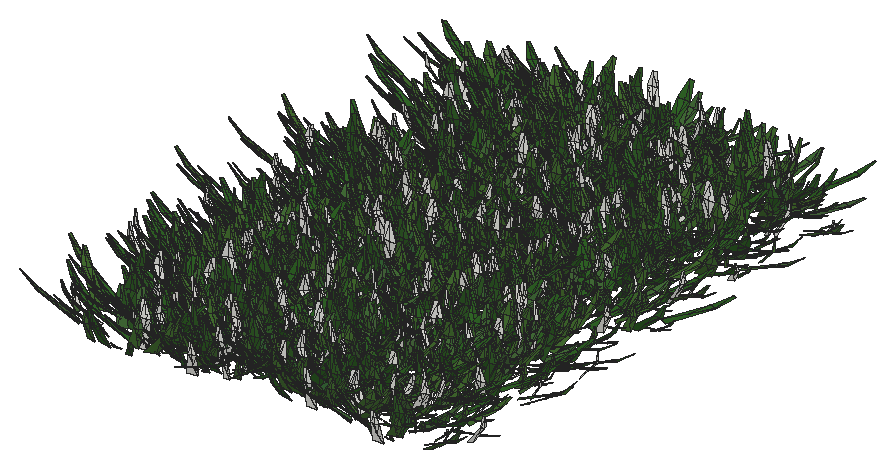
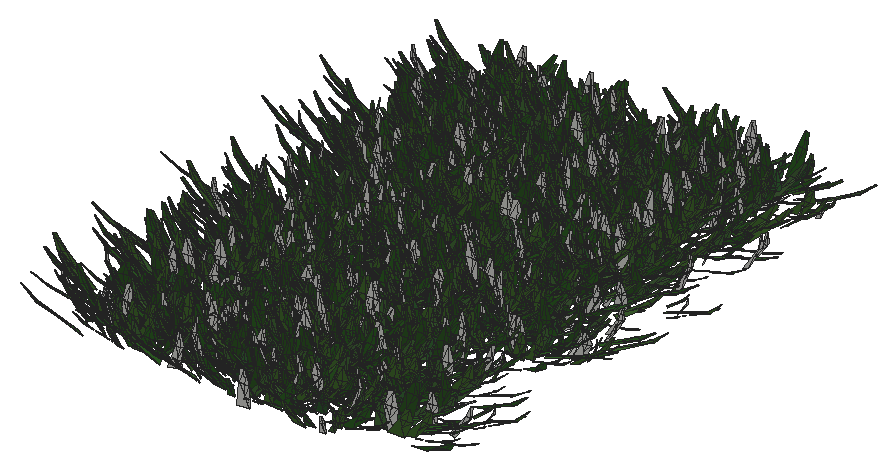
# SketchUp Ruby script. Lengths in inches.
U = 1.inch
M = Sketchup.active_model
def pt(a) = Geom::Point3d.new(a.map { |v| v * U })
def face(e, loops, mat)
  f = e.add_face(loops[0].map { |a| pt(a) })
  loops[1..].each { |l| e.add_face(l.map { |a| pt(a) }).erase! }
  f.material = f.back_material = mat if mat
  f
end
# faces: each face lists its corners as indices into pts; further lists are holes
def faces(e, pts, list, mat = nil) = list.each { |f| face(e, (f[0].is_a?(Array) ? f : [f]).map { |l| l.map { |i| pts[i] } }, mat) }
# xy, xz, yz: faces in a plane at the given z, y or x. An outline is a flat list of corners, or four numbers for a rectangle; further outlines are holes
def ring(l) = l.size == 4 ? [[l[0], l[1]], [l[2], l[1]], [l[2], l[3]], [l[0], l[3]]] : l.each_slice(2).to_a
def flat(e, list, mat, &to3) = list.each { |f| face(e, (f[0].is_a?(Array) ? f : [f]).map { |l| ring(l).map { |u, v| to3.(u, v) } }, mat) }
def xy(e, z, list, mat = nil) = flat(e, list, mat) { |x, y| [x, y, z] }
def xz(e, y, list, mat = nil) = flat(e, list, mat) { |x, z| [x, y, z] }
def yz(e, x, list, mat = nil) = flat(e, list, mat) { |y, z| [x, y, z] }
def lines(e, pts, list) = list.each { |a, b| e.add_line(pt(pts[a]), pt(pts[b])) }
# prism: a flat outline (further loops are holes) pulled along v
def prism(e, loops, v, mat = nil)
  f = face(e, loops, mat); d = Geom::Vector3d.new(v.map { |x| x * U })
  f.pushpull(f.normal.samedirection?(d) ? d.length : -d.length)
end
def box(e, o, s, mat = nil) = prism(e, [[o, [o[0] + s[0], o[1], o[2]], [o[0] + s[0], o[1] + s[1], o[2]], [o[0], o[1] + s[1], o[2]]]], [0, 0, s[2]], mat)
def at(x, y, z, deg = 0) = Geom::Transformation.translation(pt([x, y, z])) * Geom::Transformation.rotation(ORIGIN, Z_AXIS, deg.degrees)
def axes(o, x, y, z) = Geom::Transformation.new([*x, 0, *y, 0, *z, 0, *pt(o).to_a, 1])
def part(name) = M.definitions.add(name)
# library, detail: a bought-in or finely detailed component or shape, given as its bounding box
def library(name, o, s) = part(name).tap { |d| box(d.entities, o, s) }
def detail(e, o, s) = box(e.add_group.entities, o, s)
def put(e, d, t, mat = nil) = e.add_instance(d, t).tap { |i| i.material = mat if mat }
def group(e, t, mat = nil) = e.add_group.tap { |g| g.transformation = t; g.material = mat if mat }.entities
root = M.entities
M.materials.add("Material82").color = [68, 110, 58]
M.materials.add("Material83").color = [48, 90, 38]
M.materials.add("Material84").color = [68, 110, 48]
M.materials.add("Material85").color = [48, 90, 48]
M.materials.add("Material86").color = [58, 110, 58]
M.materials.add("Material87").color = [58, 90, 38]
M.materials.add("Material88").color = [68, 100, 58]
M.materials.add("Material89").color = [48, 100, 38]
c1 = part("grass00")
p = [[-0.6875,0.15,0],[-0.56,0.08,5.52],[-0.04,0.03,2.76],[0.48,-0.02,0],[0.35,-0.02,5.52],[-0.1,-0.14,5.52],
  [-0.12,0.65,8.37],[-0.42,0.65,8.37]]
faces(c1.entities,p,[[0,1,2,3],[3,2,4],[1,5,2],[5,4,2],[1,6,5],[4,5,6],[7,6,1]])
c2 = part("Group16\#1")
put(c2.entities,c1,axes([1.44,-0.61,-0.01],[0.05352,0.12609,0],[-0.10704,0.04543,0.07239],[0.06664,-0.02828,0.11628]),"Material85")
put(c2.entities,c1,axes([0.76,-0.15,-0.01],[0.04676,0.24062,0],[-0.23162,0.04501,0.06642],[0.0652,-0.01267,0.23595]),"Material82")
put(c2.entities,c1,axes([0.79,0.01,-0.01],[-0.00606,0.34651,0],[-0.34381,-0.00602,0.0432],[0.04319,0.00076,0.34386]))
put(c2.entities,c1,axes([1,0.23,-0.01],[-0.07192,0.31144,0],[-0.28722,-0.06632,0.1236],[0.12043,0.02781,0.29478]),"Material84")
put(c2.entities,c1,axes([1.66,0.77,-0.01],[-0.13828,0.29651,0],[-0.21551,-0.1005,0.22471],[0.20365,0.09498,0.23779]),"Material89")
put(c2.entities,c1,axes([0.6875,0.52,-0.01],[-0.18126,0.24051,0],[-0.22746,-0.17142,0.09788],[0.07817,0.05891,0.28481]),"Material84")
put(c2.entities,c1,axes([0.68,0.78,-0.01],[-0.215,0.18688,0],[-0.12385,-0.14248,0.21334],[0.13995,0.16101,0.18878]),"Material82")
put(c2.entities,c1,axes([0.56,1,-0.01],[-0.13756,0.07624,0],[-0.06159,-0.11112,0.0927],[0.04494,0.08108,0.12705]),"Material84")
put(c2.entities,c1,axes([0.2,0.64,-0.01],[-0.23729,0.07254,0],[-0.05711,-0.18681,0.153],[0.04473,0.14632,0.19535]),"Material89")
put(c2.entities,c1,axes([0.0625,0.72,-0.01],[-0.28874,0.02525,0],[-0.02179,-0.24916,0.14647],[0.01276,0.14591,0.25012]),"Material82")
put(c2.entities,c1,axes([-0.08,0.62,-0.01],[-0.34089,-0.04187,0],[0.03255,-0.26504,0.216],[-0.02633,0.21439,0.26703]),"Material89")
put(c2.entities,c1,axes([-0.34,0.98,-0.01],[-0.14314,-0.0493,0],[0.04397,-0.12769,0.06843],[-0.02228,0.0647,0.13505]),"Material89")
put(c2.entities,c1,axes([-0.87,1.45,-0.01],[-0.23488,-0.14114,0],[0.13761,-0.22901,0.06087],[-0.03135,0.05217,0.26717]))
put(c2.entities,c1,axes([-0.72,0.77,-0.01],[-0.14208,-0.13251,0],[0.07209,-0.0773,0.16301],[-0.11118,0.11922,0.1057]),"Material89")
put(c2.entities,c1,axes([-0.62,0.43,-0.01],[-0.14845,-0.21203,0],[0.18654,-0.13061,0.12304],[-0.10079,0.07057,0.22772]),"Material82")
put(c2.entities,c1,axes([-0.68,0.29,-0.01],[-0.13639,-0.32136,0],[0.31723,-0.13464,0.05579],[-0.05136,0.0218,0.34462]),"Material83")
put(c2.entities,c1,axes([-0.64,0.125,-0.01],[-0.0458,-0.23569,0],[0.22124,-0.043,0.08276],[-0.08124,0.01579,0.22538]),"Material86")
put(c2.entities,c1,axes([-1.6,-0.03,-0.01],[0.00576,-0.32897,0],[0.27526,0.00482,0.18018],[-0.18015,-0.00315,0.2753]),"Material84")
put(c2.entities,c1,axes([-1.36,-0.31,-0.01],[0.05718,-0.24765,0],[0.18172,0.04196,0.17267],[-0.16825,-0.03885,0.1865]),"Material89")
put(c2.entities,c1,axes([-1.54,-0.72,-0.01],[0.06537,-0.14017,0],[0.13555,0.06321,0.03939],[-0.0357,-0.01665,0.14956]))
put(c2.entities,c1,axes([-1.19,-0.9,-0.01],[0.09597,-0.12735,0],[0.11214,0.08451,0.07557],[-0.06035,-0.04548,0.14042]),"Material88")
put(c2.entities,c1,axes([-0.47,-0.54,-0.01],[0.11588,-0.10072,0],[0.0618,0.0711,0.12124],[-0.07953,-0.0915,0.0942]))
put(c2.entities,c1,axes([-0.47,-0.84,-0.01],[0.11927,-0.0661,0],[0.06603,0.11913,0.00646],[-0.00313,-0.00565,0.13621]),"Material84")
put(c2.entities,c1,axes([-0.38,-1.24,-0.01],[0.28037,-0.08571,0],[0.0618,0.20215,0.20315],[-0.05939,-0.19428,0.21139]),"Material88")
put(c2.entities,c1,axes([-0.06,-0.66,-0.01],[0.22719,-0.01987,0],[0.01247,0.14255,0.17758],[-0.01547,-0.17691,0.1431]),"Material87")
put(c2.entities,c1,axes([0.11,-0.89,-0.01],[0.14882,0.01828,0],[-0.01058,0.08611,0.12229],[0.01491,-0.12138,0.08676]),"Material85")
put(c2.entities,c1,axes([0.25,-0.72,-0.01],[0.20481,0.07053,0],[-0.06206,0.18022,0.10291],[0.03351,-0.0973,0.1906]),"Material85")
put(c2.entities,c1,axes([0.85,-1.42,-0.01],[0.16481,0.09904,0],[-0.09472,0.15762,0.05616],[0.02893,-0.04814,0.18389]),"Material84")
put(c2.entities,c1,axes([1.01,-1.09,-0.01],[0.21858,0.20385,0],[-0.17495,0.1876,0.15339],[0.10462,-0.11218,0.25652]),"Material89")
put(c2.entities,c1,axes([1.01,-0.71,-0.01],[0.08733,0.12473,0],[-0.06445,0.04512,0.13037],[0.1068,-0.07477,0.07867]),"Material85")
c3 = part("Group15\#1")
put(c3.entities,c2,at(0,0,0))
c4 = part("3darcstudiotree_grass00\#1")
put(c4.entities,c3,at(0,0,0))
put(root,c4,axes([778.4,976.55,-29.74],[-0.54088,1.62044,0],[-3.31155,-0.17191,-0.03263],[-0.19335,-0.01004,1.49628]))
put(root,c4,axes([778.59,975.01,-29.74],[3.70566,-0.42814,0],[1.15173,1.5504,-0.01036],[0.01836,0.02471,1.93559]))
put(root,c4,axes([779.09,940.33,-29.74],[2.92691,-1.3802,0],[3.11862,1.02859,-0.02296],[0.10607,0.03499,1.8355]))
put(root,c4,axes([778.89,994.31,-29.74],[-0.97344,1.33602,0],[-4.5066,-0.51069,-0.06106],[-0.24596,-0.02787,1.47293]))
put(root,c4,axes([778.71,963.53,-29.74],[4.64499,-0.27977,0],[0.53132,1.372,-0.02943],[0.02555,0.06597,1.51666]))
put(root,c4,axes([780.17,961.14,-29.74],[-0.18207,-1.50592,0],[4.09357,-0.07698,-0.05646],[0.28834,-0.00542,1.57058]))
put(root,c4,axes([778.84,950.76,-29.74],[2.47814,1.17598,0],[-3.14029,1.02922,-0.05468],[-0.21842,0.07159,1.58958]))
put(root,c4,axes([778.81,973.05,-29.74],[4.42055,0.62646,0],[-1.4719,1.61538,-0.03831],[-0.06085,0.06679,1.53223]))
put(root,c4,axes([779.33,989.9,-29.74],[4.51641,-0.1704,0],[0.33815,1.39393,-0.00501],[0.00291,0.012,1.62495]))
put(root,c4,axes([779.03,952.9375,-29.74],[2.33395,1.59128,0],[-3.69314,0.84246,-0.02506],[-0.12399,0.02828,1.82822]))
put(root,c4,axes([779.62,944.71,-29.74],[3.72841,-0.11021,0],[0.34874,1.83494,-0.00347],[0.00143,0.00753,1.92949]))
put(root,c4,axes([780.61,986.01,-29.74],[-2.15234,1.14546,0],[-3.3995,-0.99347,-0.05517],[-0.2418,-0.07066,1.72999]))
put(root,c4,axes([779.91,959.73,-29.74],[2.3917,1.38211,0],[-2.775,0.74686,-0.01403],[-0.09111,0.02452,1.97952]))
put(root,c4,axes([780.01,968.4,-29.74],[3.05644,0.96272,0],[-2.54771,1.25799,-0.04015],[-0.1144,0.05649,1.39698]))
put(root,c4,axes([780.57,955.42,-29.74],[0.44258,1.4547,0],[-3.4051,0.16112,-0.01784],[-0.12417,0.00588,1.80168]))
put(root,c4,axes([782.2,982.97,-29.74],[-1.45799,-1.43911,0],[3.11235,-0.49041,-0.01431],[0.09188,-0.01448,1.73701]))
put(root,c4,axes([782.36,942.56,-29.74],[-2.77273,1.25915,0],[-2.61353,-0.89509,-0.01448],[-0.05898,-0.0202,1.39954]))
put(root,c4,axes([783.32,944.09,-29.74],[-3.67224,-0.62774,0],[1.3268,-1.20717,-0.04544],[0.10775,-0.09803,1.4908]))
put(root,c4,axes([783.58,976.69,-29.74],[-4.47177,0.4092,0],[-0.80597,-1.36984,-0.03599],[-0.04373,-0.07433,1.43677]))
put(root,c4,axes([782.96,954.99,-29.74],[-3.07968,1.30519,0],[-3.32937,-1.22181,-0.01383],[-0.04412,-0.01619,1.48532]))
put(root,c4,axes([782.5,966.41,-29.74],[3.91717,0.58785,0],[-1.40512,1.45623,-0.01203],[-0.02325,0.0241,1.60927]))
put(root,c4,axes([784.36,961.55,-29.74],[-1.04981,-1.26066,0],[3.51989,-0.45588,-0.02104],[0.10484,-0.01358,1.45661]))
put(root,c4,axes([783.63,958.11,-29.74],[3.15172,-0.92963,0],[2.70365,1.42561,-0.02614],[0.06865,0.0362,1.48366]))
put(root,c4,axes([784.4,964.35,-29.74],[-4.56421,0.17831,0],[-0.33265,-1.32435,-0.0174],[-0.0117,-0.04658,1.72585]))
put(root,c4,axes([784.89,990.04,-29.74],[-3.08784,-0.53374,0],[1.78756,-1.6084,-0.00176],[0.00414,-0.00372,1.95594]))
put(root,c4,axes([783.95,950.46,-29.74],[-2.14552,1.35971,0],[-3.80804,-0.93454,-0.04897],[-0.2422,-0.05944,1.9584]))
put(root,c4,axes([783.41,947.17,-29.74],[3.03533,0.518,0],[-1.31858,1.2017,-0.02703],[-0.08286,0.07551,1.9211]))
put(root,c4,axes([785.25,972.37,-29.74],[-2.79081,-0.68685,0],[2.20267,-1.39196,-0.00523],[0.01654,-0.01045,1.86317]))
put(root,c4,axes([785.38,975.79,-29.74],[-3.42781,-0.73376,0],[1.91044,-1.38806,-0.04387],[0.11882,-0.08633,1.70431]))
put(root,c4,axes([784.6875,948.51,-29.74],[-3.41152,0.77464,0],[-2.34689,-1.60751,-0.0199],[-0.0471,-0.03226,1.67187]))
put(root,c4,axes([783.69,971.16,-29.74],[1.53269,1.16919,0],[-3.90157,0.79546,-0.03477],[-0.15934,0.03249,1.69826]))
put(root,c4,axes([784.98,959.12,-29.74],[-2.82754,1.11661,0],[-2.90837,-1.14544,-0.05526],[-0.21558,-0.0849,1.69871]))
put(root,c4,axes([784.99,952.53,-29.74],[2.39859,-1.38317,0],[2.89597,0.78107,-0.02882],[0.1286,0.03468,1.42183]))
put(root,c4,axes([785.42,996.9375,-29.74],[0.37671,-1.60669,0],[3.58296,0.13066,-0.04487],[0.23434,0.00855,1.41449]))
put(root,c4,axes([785.83,995.4375,-29.74],[-4.41181,-0.09171,0],[0.23476,-1.75641,-0.0488],[0.01273,-0.09527,1.65721]))
put(root,c4,axes([785.69,940.76,-29.74],[-3.47293,0.19496,0],[-0.50842,-1.40863,-0.03826],[-0.03299,-0.09141,1.65468]))
put(root,c4,axes([786.25,991.8,-29.74],[-4.2727,-0.29638,0],[0.78575,-1.76178,-0.04722],[0.03378,-0.07573,1.40384]))
put(root,c4,axes([784.9,987.32,-29.74],[-0.9668,1.66725,0],[-3.92404,-0.3539,-0.0233],[-0.11915,-0.01075,1.58282]))
put(root,c4,axes([784.95,968.64,-29.74],[3.78841,0.96012,0],[-2.55963,1.5708,-0.03131],[-0.07104,0.04359,1.48921]))
put(root,c4,axes([785.2,981.64,-29.74],[2.7139,1.45109,0],[-3.63417,1.0571,-0.05484],[-0.17137,0.04985,1.31443]))
put(root,c4,axes([785.76,979.63,-29.74],[3.41186,0.04199,0],[-0.11049,1.39641,-0.01718],[-0.0038,0.04797,1.88076]))
put(root,c4,axes([787.83,958.1,-29.74],[-3.09292,-0.92086,0],[2.57207,-1.3436,-0.01411],[0.04505,-0.02353,1.69584]))
put(root,c4,axes([785.99,985.4,-29.74],[0.1551,1.54916,0],[-4.73746,0.07377,-0.04149],[-0.18002,0.0028,1.54325]))
put(root,c4,axes([788.01,976.88,-29.74],[0.67498,-1.80639,0],[4.18251,0.24307,-0.00777],[0.03281,0.00191,1.3523]))
put(root,c4,axes([788.18,972.86,-29.74],[-0.75947,-1.30953,0],[4.19896,-0.37875,-0.04627],[0.26037,-0.02349,1.86363]))
put(root,c4,axes([788.22,959.17,-29.74],[-4.1346,0.13575,0],[-0.2838,-1.34436,-0.02559],[-0.01617,-0.0766,1.95328]))
put(root,c4,axes([788.99,970.48,-29.74],[1.00092,-1.32759,0],[4.42574,0.51896,-0.06029],[0.29852,0.035,1.78762]))
put(root,c4,axes([788.69,991.66,-29.74],[2.10537,-1.23806,0],[3.71835,0.98344,-0.05795],[0.27877,0.07373,1.94389]))
put(root,c4,axes([788.04,946.54,-29.74],[3.79547,0.16316,0],[-0.37027,1.33962,-0.03498],[-0.02197,0.07948,1.48455]))
put(root,c4,axes([788.89,966.05,-29.74],[-3.00276,0.99555,0],[-2.11915,-0.9941,-0.00081],[-0.00373,-0.00175,1.76997]))
put(root,c4,axes([790.01,984.25,-29.74],[-0.04764,-1.42757,0],[4.50476,-0.02338,-0.00745],[0.04284,-0.00022,1.94284]))
put(root,c4,axes([788.7,942.28,-29.74],[0.27257,1.5962,0],[-3.57048,0.09483,-0.04154],[-0.28788,0.00765,1.86323]))
put(root,c4,axes([790.15,979.48,-29.74],[-4.51182,-0.35471,0],[0.87439,-1.72977,-0.01918],[0.02129,-0.04212,1.90358]))
put(root,c4,axes([788.92,986.4375,-29.74],[2.9902,-0.77103,0],[1.83544,1.10708,-0.045],[0.13449,0.08112,1.37282]))
put(root,c4,axes([790.19,964.39,-29.74],[0.52861,-1.48035,0],[4.44113,0.24665,-0.00524],[0.03043,0.00169,1.97007]))
put(root,c4,axes([788.49,953.83,-29.74],[1.62026,1.14881,0],[-2.90984,0.63829,-0.00131],[-0.00892,0.00196,1.9458]))
put(root,c4,axes([789.51,944.28,-29.74],[-3.07094,0.93295,0],[-2.23562,-1.14452,-0.00087],[-0.00325,-0.00166,1.68429]))
put(root,c4,axes([790.56,950.63,-29.74],[-1.32818,-1.26932,0],[4.11875,-0.67029,-0.01762],[0.07227,-0.01176,1.48208]))
put(root,c4,axes([788.65,948.25,-29.74],[3.48613,0.95688,0],[-2.23612,1.26704,-0.01513],[-0.04219,0.02391,1.43215]))
put(root,c4,axes([789.73,981.34,-29.74],[3.73229,-0.67208,0],[1.78653,1.54305,-0.05401],[0.10032,0.08665,1.44188]))
put(root,c4,axes([791.38,994.4375,-29.74],[-3.64932,-0.7532,0],[1.94147,-1.463,-0.05348],[0.14522,-0.10943,1.83786]))
put(root,c4,axes([790.08,968.61,-29.74],[4.39358,-0.14103,0],[0.35283,1.70956,-0.02372],[0.00876,0.04243,1.48337]))
put(root,c4,axes([791.57,996.02,-29.74],[-4.22243,0.41861,0],[-0.86072,-1.35028,-0.03206],[-0.04838,-0.0759,1.63785]))
put(root,c4,axes([790.59,987.81,-29.74],[2.4549,0.99675,0],[-3.14112,1.20322,-0.03466],[-0.14383,0.05509,1.89896]))
put(root,c4,axes([790.64,974.69,-29.74],[3.48474,0.89145,0],[-2.45497,1.49256,-0.05832],[-0.13986,0.08503,1.48992]))
put(root,c4,axes([791.17,990.48,-29.74],[-0.03901,1.43427,0],[-3.74587,-0.01585,-0.03184],[-0.19446,-0.00082,1.71482]))
put(root,c4,axes([791.55,962.16,-29.74],[-1.95042,1.47202,0],[-4.16072,-0.85742,-0.06253],[-0.2988,-0.06158,1.89715]))
put(root,c4,axes([791.45,955.55,-29.74],[3.54296,-0.10072,0],[0.24357,1.33252,-0.00836],[0.00467,0.02557,1.97523]))
put(root,c4,axes([793.65,972.91,-29.74],[-3.58618,-0.76762,0],[2.12856,-1.54662,-0.04044],[0.10752,-0.07813,1.86421]))
put(root,c4,axes([793.93,968.36,-29.74],[-3.71376,-0.4791,0],[1.06109,-1.27925,-0.035],[0.07367,-0.08882,1.73222]))
put(root,c4,axes([794.48,988.51,-29.74],[-3.76687,-0.82913,0],[2.27178,-1.60524,-0.0179],[0.04066,-0.02873,1.62858]))
put(root,c4,axes([793.64,950.84,-29.74],[-3.28554,0.84585,0],[-2.43757,-1.4726,-0.04574],[-0.1384,-0.08361,1.85022]))
put(root,c4,axes([794.39,949.5,-29.74],[0.43132,-1.66774,0],[3.95027,0.1589,-0.00761],[0.04938,0.00199,1.94156]))
put(root,c4,axes([794.65,976.58,-29.74],[-3.03865,-1.23581,0],[2.76731,-1.05827,-0.04714],[0.18592,-0.0711,1.58733]))
put(root,c4,axes([793.23,945.875,-29.74],[4.71636,-0.1967,0],[0.48906,1.82382,-0.02611],[0.01545,0.05763,1.96192]))
put(root,c4,axes([794.33,979.12,-29.74],[-3.07129,1.23004,0],[-2.90171,-1.12685,-0.02428],[-0.07533,-0.02925,1.32917]))
put(root,c4,axes([795.24,953.86,-29.74],[-3.14124,-0.52931,0],[1.80451,-1.66556,-0.04539],[0.09971,-0.09203,1.92461]))
put(root,c4,axes([793.96,997.4,-29.74],[4.37264,-0.16186,0],[0.38997,1.63854,-0.03728],[0.02119,0.08905,1.90298]))
put(root,c4,axes([794.3,991.83,-29.74],[4.22982,-0.69798,0],[1.45654,1.37281,-0.04818],[0.09708,0.0915,1.47658]))
put(root,c4,axes([794.5625,990.87,-29.74],[3.5272,-0.10967,0],[0.36977,1.84972,-0.03935],[0.01267,0.0634,1.44542]))
put(root,c4,axes([795.3,983.14,-29.74],[2.22522,-0.98382,0],[3.26699,1.14926,-0.04874],[0.15967,0.05617,1.44038]))
put(root,c4,axes([794.5,957.58,-29.74],[4.40761,-0.00182,0],[0.00468,1.76466,-0.04894],[0.00022,0.08123,1.41164]))
put(root,c4,axes([796.39,975.77,-29.74],[-3.1255,-0.93872,0],[2.35839,-1.22127,-0.01582],[0.04515,-0.02338,1.37394]))
put(root,c4,axes([795.35,971.33,-29.74],[-2.15998,1.50569,0],[-3.5128,-0.78375,-0.02589],[-0.10439,-0.02329,1.40149]))
put(root,c4,axes([795.83,994.6875,-29.74],[2.50422,-1.12718,0],[2.64209,0.91293,-0.00209],[0.0092,0.00318,1.54397]))
put(root,c4,axes([795.99,986.33,-29.74],[-3.79899,1.04858,0],[-2.13311,-1.20197,-0.01309],[-0.05055,-0.02848,1.87779]))
put(root,c4,axes([796.66,956.11,-29.74],[-0.77442,-1.59147,0],[3.42237,-0.25901,-0.00431],[0.02185,-0.00165,1.34772]))
put(root,c4,axes([796.9375,942.86,-29.74],[-1.56215,-1.16443,0],[3.47638,-0.72535,-0.0302],[0.1517,-0.03165,1.67548]))
put(root,c4,axes([797.02,961.6,-29.74],[0.16922,-1.40325,0],[3.56749,0.06691,-0.0123],[0.08099,0.00152,1.7643]))
put(root,c4,axes([795.84,965.91,-29.74],[3.21803,0.34517,0],[-1.06694,1.54707,-0.02379],[-0.03071,0.04453,1.49895]))
put(root,c4,axes([795.6,959.62,-29.74],[1.18275,1.22871,0],[-4.35683,0.65227,-0.02635],[-0.11985,0.01794,1.69955]))
put(root,c4,axes([797.27,981.5,-29.74],[-4.55654,0.30056,0],[-0.72952,-1.72007,-0.00717],[-0.00538,-0.01268,1.50735]))
put(root,c4,axes([796.76,964.58,-29.74],[2.66801,-0.76193,0],[2.24823,1.2244,-0.04376],[0.15596,0.08494,1.7457]))
put(root,c4,axes([798.85,972.15,-29.74],[-2.4386,-1.43306,0],[3.07254,-0.81318,-0.00883],[0.05033,-0.01332,1.90461]))
put(root,c4,axes([799.23,990.58,-29.74],[-2.69612,-1.17454,0],[3.29179,-1.17522,-0.01753],[0.05781,-0.02064,1.48083]))
put(root,c4,axes([797.1875,944.46,-29.74],[-0.169,1.77802,0],[-4.32571,-0.06395,-0.00219],[-0.00941,-0.00014,1.39308]))
put(root,c4,axes([799.42,948.11,-29.74],[-3.83813,-1.06248,0],[2.06139,-1.15817,-0.02484],[0.08815,-0.04953,1.66133]))
put(root,c4,axes([799.11,984.43,-29.74],[-4.08007,0.11151,0],[-0.22831,-1.29918,-0.01842],[-0.00694,-0.03947,1.34789]))
put(root,c4,axes([799.6,942.67,-29.74],[-3.13096,0.65051,0],[-1.62991,-1.22011,-0.01732],[-0.0588,-0.04402,1.90951]))
put(root,c4,axes([800.8,995.01,-29.74],[-1.34356,-1.54381,0],[4.22745,-0.57221,-0.00214],[0.01038,-0.00141,1.72072]))
put(root,c4,axes([798.86,950.22,-29.74],[3.83567,0.80348,0],[-1.71741,1.27513,-0.04207],[-0.13622,0.10114,1.89419]))
put(root,c4,axes([799.29,966.3125,-29.74],[2.14752,1.24419,0],[-2.84206,0.76295,-0.02533],[-0.12904,0.03464,1.58831]))
put(root,c4,axes([799.89,988.64,-29.74],[4.00755,-0.76372,0],[1.77132,1.44561,-0.00312],[0.00773,0.00631,1.73901]))
put(root,c4,axes([799.59,959.82,-29.74],[0.92286,1.78615,0],[-4.03148,0.32396,-0.0503],[-0.25163,0.02022,1.57458]))
put(root,c4,axes([799.92,974.88,-29.74],[-1.5079,1.48015,0],[-3.78766,-0.60014,-0.02547],[-0.10708,-0.01697,1.38631]))
put(root,c4,axes([800.97,956.86,-29.74],[0.88426,-1.72062,0],[4.38154,0.35021,-0.041],[0.21175,0.01693,1.76588]))
put(root,c4,axes([799.79,952.75,-29.74],[4.1439,0.48612,0],[-1.21296,1.60815,-0.03162],[-0.038,0.05038,1.3441]))
put(root,c4,axes([799.65,967.88,-29.74],[2.12924,1.06786,0],[-3.55371,1.10206,-0.01217],[-0.05143,0.01595,1.82194]))
put(root,c4,axes([801.22,943.78,-29.74],[1.5808,-1.43275,0],[3.65536,0.62726,-0.04597],[0.19603,0.03364,1.38947]))
put(root,c4,axes([802.11,947.09,-29.74],[-4.27451,-0.64112,0],[1.27307,-1.32012,-0.04106],[0.09351,-0.09696,1.71966]))
put(root,c4,axes([802.04,992.01,-29.74],[-3.75297,0.08152,0],[-0.23562,-1.68719,-0.02509],[-0.00578,-0.04142,1.34616]))
put(root,c4,axes([802.68,982.35,-29.74],[-0.74737,-1.75822,0],[4.00395,-0.2647,-0.02808],[0.1526,-0.01009,1.67665]))
put(root,c4,axes([801.93,963.58,-29.74],[2.37533,-1.57622,0],[3.03149,0.71052,-0.0411],[0.20378,0.04776,1.52451]))
put(root,c4,axes([801.13,977.06,-29.74],[3.22242,0.46316,0],[-1.61234,1.7447,-0.03532],[-0.06153,0.06658,1.79519]))
put(root,c4,axes([801.62,971.43,-29.74],[0.53134,1.4221,0],[-3.42638,0.19911,-0.04131],[-0.21204,0.01232,1.34689]))
put(root,c4,axes([802.1,962.64,-29.74],[3.9417,-1.03975,0],[1.84996,1.09076,-0.03191],[0.12762,0.07525,1.79443]))
put(root,c4,axes([802.49,955.36,-29.74],[3.56947,-0.45549,0],[1.31887,1.60745,-0.01717],[0.02449,0.02985,1.48777]))
put(root,c4,axes([802.57,978.75,-29.74],[0.55525,1.71346,0],[-3.482,0.17549,-0.04145],[-0.30813,0.01553,1.97198]))
put(root,c4,axes([802.32,985.74,-29.74],[3.66484,0.89609,0],[-2.00603,1.27601,-0.03504],[-0.12347,0.07854,1.90819]))
put(root,c4,axes([804.53,948.68,-29.74],[-1.10349,-1.4395,0],[4.41957,-0.52692,-0.03772],[0.14279,-0.01702,1.36861]))
put(root,c4,axes([804.32,978.59,-29.74],[-2.20687,1.14075,0],[-3.09016,-0.92978,-0.05103],[-0.23957,-0.07208,1.72023]))
put(root,c4,axes([804.79,990.62,-29.74],[-3.32366,1.12138,0],[-2.70082,-1.24501,-0.05065],[-0.15287,-0.07047,1.44592]))
put(root,c4,axes([805.875,975.37,-29.74],[-2.7638,-1.30283,0],[3.13183,-1.03331,-0.01878],[0.07913,-0.02611,1.68146]))
put(root,c4,axes([806.1,968.09,-29.74],[-3.16827,-0.67396,0],[1.62868,-1.19079,-0.04409],[0.1208,-0.08832,1.48398]))
put(root,c4,axes([805.86,976.43,-29.74],[-4.1698,0.79339,0],[-1.666,-1.36181,-0.02532],[-0.06287,-0.05139,1.64221]))
put(root,c4,axes([804.82,996.75,-29.74],[3.81533,0.48086,0],[-1.13696,1.40304,-0.03842],[-0.0798,0.09848,1.90991]))
put(root,c4,axes([805.43,961.15,-29.74],[3.77642,-0.7823,0],[1.66108,1.24712,-0.02304],[0.07142,0.05362,1.78453]))
put(root,c4,axes([806.96,988.36,-29.74],[0.63263,-1.77026,0],[4.09912,0.22783,-0.02402],[0.14113,0.00784,1.84088]))
put(root,c4,axes([807.1,952.63,-29.74],[-4.44839,0.03138,0],[-0.07411,-1.6342,-0.01042],[-0.00109,-0.02408,1.82123]))
put(root,c4,axes([807.08,941.76,-29.74],[-3.4085,0.44598,0],[-1.18576,-1.40948,-0.04681],[-0.08042,-0.0956,1.53984]))
put(root,c4,axes([805.84,951.4,-29.74],[3.54482,0.3991,0],[-1.20365,1.66273,-0.00872],[-0.01104,0.01525,1.51538]))
put(root,c4,axes([806.47,981.39,-29.74],[-0.28998,1.73456,0],[-3.34694,-0.08702,-0.03816],[-0.29536,-0.00768,1.95014]))
put(root,c4,axes([805.6875,946.2,-29.74],[3.41397,1.21641,0],[-2.3032,1.00536,-0.00582],[-0.0237,0.01035,1.56404]))
put(root,c4,axes([805.8125,957.63,-29.74],[2.93721,1.2592,0],[-3.10849,1.12772,-0.033],[-0.144,0.05224,1.87715]))
put(root,c4,axes([807.98,959.2,-29.74],[-1.1478,-1.40641,0],[4.093,-0.51953,-0.0477],[0.19511,-0.02477,1.385]))
put(root,c4,axes([808.37,945.06,-29.74],[-2.49924,-1.08664,0],[2.82442,-1.01033,-0.0539],[0.19999,-0.07154,1.43163]))
put(root,c4,axes([806.76,964.59,-29.74],[2.93445,0.88211,0],[-2.13254,1.10335,-0.01463],[-0.05848,0.03025,1.73802]))
put(root,c4,axes([806.875,956.09,-29.74],[3.48566,0.55514,0],[-1.55719,1.52067,-0.03343],[-0.07577,0.07399,1.88641]))
put(root,c4,axes([807.34,994.63,-29.74],[-0.15322,1.4871,0],[-3.57108,-0.05722,-0.03031],[-0.19833,-0.00318,1.75443]))
put(root,c4,axes([807.03,973.48,-29.74],[3.31433,0.47754,0],[-1.51472,1.63504,-0.04863],[-0.07862,0.08486,1.5585]))
put(root,c4,axes([808.26,993.22,-29.74],[-3.94658,0.83198,0],[-2.08533,-1.53849,-0.02635],[-0.05206,-0.03841,1.3895]))
put(root,c4,axes([806.88,985.74,-29.74],[2.20824,1.44568,0],[-4.06639,0.96604,-0.01693],[-0.06521,0.01549,1.59984]))
put(root,c4,axes([807.62,970.04,-29.74],[4.53975,0.53985,0],[-1.08694,1.4216,-0.04516],[-0.08333,0.10898,1.80387]))
put(root,c4,axes([808.33,982.97,-29.74],[-2.27595,1.46975,0],[-3.85308,-0.92798,-0.0342],[-0.14118,-0.034,1.63693]))
